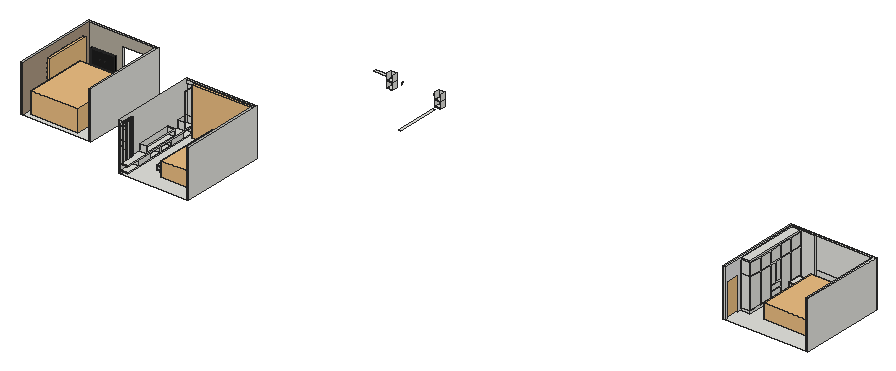
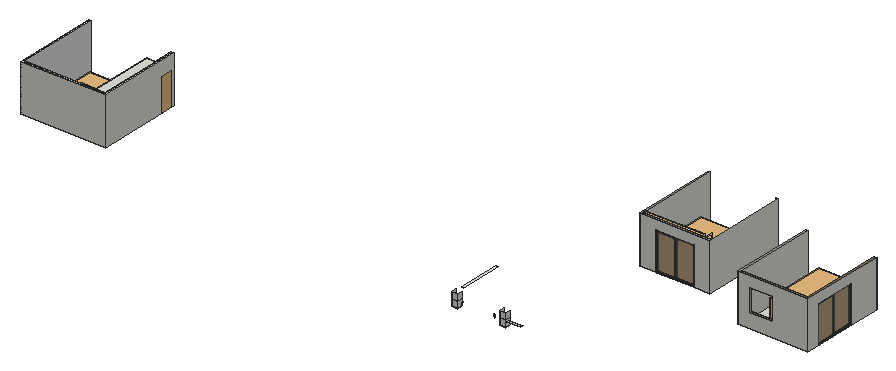
# SketchUp Ruby script. Lengths in inches.
U = 1.inch
M = Sketchup.active_model
def pt(a) = Geom::Point3d.new(a.map { |v| v * U })
def face(e, loops, mat)
  f = e.add_face(loops[0].map { |a| pt(a) })
  loops[1..].each { |l| e.add_face(l.map { |a| pt(a) }).erase! }
  f.material = f.back_material = mat if mat
  f
end
# faces: each face lists its corners as indices into pts; further lists are holes
def faces(e, pts, list, mat = nil) = list.each { |f| face(e, (f[0].is_a?(Array) ? f : [f]).map { |l| l.map { |i| pts[i] } }, mat) }
# xy, xz, yz: faces in a plane at the given z, y or x. An outline is a flat list of corners, or four numbers for a rectangle; further outlines are holes
def ring(l) = l.size == 4 ? [[l[0], l[1]], [l[2], l[1]], [l[2], l[3]], [l[0], l[3]]] : l.each_slice(2).to_a
def flat(e, list, mat, &to3) = list.each { |f| face(e, (f[0].is_a?(Array) ? f : [f]).map { |l| ring(l).map { |u, v| to3.(u, v) } }, mat) }
def xy(e, z, list, mat = nil) = flat(e, list, mat) { |x, y| [x, y, z] }
def xz(e, y, list, mat = nil) = flat(e, list, mat) { |x, z| [x, y, z] }
def yz(e, x, list, mat = nil) = flat(e, list, mat) { |y, z| [x, y, z] }
def lines(e, pts, list) = list.each { |a, b| e.add_line(pt(pts[a]), pt(pts[b])) }
# prism: a flat outline (further loops are holes) pulled along v
def prism(e, loops, v, mat = nil)
  f = face(e, loops, mat); d = Geom::Vector3d.new(v.map { |x| x * U })
  f.pushpull(f.normal.samedirection?(d) ? d.length : -d.length)
end
def box(e, o, s, mat = nil) = prism(e, [[o, [o[0] + s[0], o[1], o[2]], [o[0] + s[0], o[1] + s[1], o[2]], [o[0], o[1] + s[1], o[2]]]], [0, 0, s[2]], mat)
def at(x, y, z, deg = 0) = Geom::Transformation.translation(pt([x, y, z])) * Geom::Transformation.rotation(ORIGIN, Z_AXIS, deg.degrees)
def axes(o, x, y, z) = Geom::Transformation.new([*x, 0, *y, 0, *z, 0, *pt(o).to_a, 1])
def part(name) = M.definitions.add(name)
# library, detail: a bought-in or finely detailed component or shape, given as its bounding box
def library(name, o, s) = part(name).tap { |d| box(d.entities, o, s) }
def detail(e, o, s) = box(e.add_group.entities, o, s)
def put(e, d, t, mat = nil) = e.add_instance(d, t).tap { |i| i.material = mat if mat }
def group(e, t, mat = nil) = e.add_group.tap { |g| g.transformation = t; g.material = mat if mat }.entities
root = M.entities
M.materials.add("[0135_DarkGray]").color = [81, 81, 81]
M.materials.add("[Color_001]").color = [226, 226, 226]
M.materials.add("[Color_007]").color = [58, 58, 58]
M.materials.add("[Color_009]").color = [0, 0, 0]
M.materials.add("[Color_B19]").color = [180, 172, 158]
M.materials.add("[Color_D14]").color = [173, 154, 131]
M.materials.add("[Translucent Glass Gray]").color = [128, 128, 128]
M.materials["[Translucent Glass Gray]"].alpha = 0.15
M.materials.add("blackened steel1").color = [30, 30, 30]
c1 = library("bed",[-25.65,-58.99,0],[75.48,89.46,37.24])
c2 = library("Garniza_zaclona\#2",[1.52,0,0],[127.96,8.15,78.72])
c3 = part("PENTEK_RP Fineline 50S_SlidingDoor_GlazingBead_2")
box(c3.entities,[0,0,0],[0.56,0.59,94.39],"[0135_DarkGray]")
c4 = part("PENTEK_RP Fineline 50S_SlidingDoor_Glass")
box(c4.entities,[0,0,0],[46.58,0.16,94.39],"[Translucent Glass Gray]")
c5 = part("PENTEK_RP Fineline 50S_SlidingDoor_GlazingBead")
box(c5.entities,[0,0,0],[45.47,0.59,0.56],"[0135_DarkGray]")
c6 = part("PENTEK_RP Fineline 50S_SlidingDoor_Leaf_E1")
xy(c6.entities,0,[[0,0,0.93,1.97],[0.93,1.57,1.49,1.97]],"[0135_DarkGray]")
xy(c6.entities,96.25,[[0,0,0.93,0,0.93,1.57,1.49,1.57,1.49,1.97,0,1.97]],"[0135_DarkGray]")
xz(c6.entities,0,[[0,0,0.93,96.25]],"[0135_DarkGray]")
xz(c6.entities,1.57,[[0.93,0,1.49,95.32],[0.93,95.32,1.49,96.25]],"[0135_DarkGray]")
xz(c6.entities,1.97,[[0,0,1.49,96.25]],"[0135_DarkGray]")
yz(c6.entities,0,[[0,0,1.97,96.25]],"[0135_DarkGray]")
yz(c6.entities,0.93,[[0,0,1.57,0.93],[0,0.93,1.57,95.32],[0,95.32,1.57,96.25]],"[0135_DarkGray]")
yz(c6.entities,1.49,[[1.57,0,1.97,95.32],[1.57,95.32,1.97,96.25]],"[0135_DarkGray]")
c7 = part("PENTEK_RP Fineline 50S_SlidingDoor_Leaf_E2")
xy(c7.entities,0,[[0,0,0,1.57,0.56,1.57,0.56,1.97,46.02,1.97,46.02,1.57,46.58,1.57,46.58,0]],"[0135_DarkGray]")
xy(c7.entities,0.93,[[0,0,46.58,1.57]],"[0135_DarkGray]")
xy(c7.entities,1.49,[[0.56,1.57,46.02,1.97]],"[0135_DarkGray]")
xz(c7.entities,0,[[0,0,46.58,0.93]],"[0135_DarkGray]")
xz(c7.entities,1.57,[[0,0,0.56,0.93],[46.02,0,46.58,0.93],[0.56,0.93,46.02,1.49]],"[0135_DarkGray]")
xz(c7.entities,1.97,[[0.56,0,46.02,1.49]],"[0135_DarkGray]")
yz(c7.entities,0,[[0,0,1.57,0.93]],"[0135_DarkGray]")
yz(c7.entities,0.56,[[1.57,0,1.97,0.93],[1.57,0.93,1.97,1.49]],"[0135_DarkGray]")
yz(c7.entities,46.02,[[1.57,0,1.97,0.93],[1.57,0.93,1.97,1.49]],"[0135_DarkGray]")
yz(c7.entities,46.58,[[0,0,1.57,0.93]],"[0135_DarkGray]")
c8 = part("PENTEK_RP Fineline S_SlidingDoor_Leaf1")
put(c8.entities,c3,at(0.93,0,0.93))
put(c8.entities,c3,at(46.96,0,0.93))
put(c8.entities,c4,at(1.49,1.42,0.93))
put(c8.entities,c5,at(1.49,0,0.93))
put(c8.entities,c4,at(1.49,0.59,0.93))
put(c8.entities,c6,at(0,0,0))
put(c8.entities,c6,axes([48.44,0,0],[-1,0,0],[0,1,0],[0,0,1]))
put(c8.entities,c7,axes([0.93,0,96.25],[1,0,0],[0,1,0],[0,0,-1]))
put(c8.entities,c7,at(0.93,0,0))
put(c8.entities,c5,at(1.49,0,94.77))
c9 = part("PENTEK_RP Fineline 50S_Sliding_DoorCase_E1")
box(c9.entities,[0,0,0],[1.51,3.66,99.27],"[0135_DarkGray]")
c10 = part("PENTEK_RP Fineline 50S_SlidingDooe_Case_E2")
box(c10.entities,[0,0,0],[96.25,3.66,1.51],"[0135_DarkGray]")
c11 = part("pentek_RP Fineline 50S_SlidingDoor_Case")
put(c11.entities,c9,at(97.76,0,0))
put(c11.entities,c10,at(1.51,0,0))
put(c11.entities,c9,at(0,0,0))
put(c11.entities,c10,at(1.51,0,97.76))
c12 = part("PENTEK_RP Fineline 50S_SlidingDoor_Leaf2")
put(c12.entities,c4,at(1.49,1.42,0.93))
put(c12.entities,c5,at(1.49,0,94.77))
put(c12.entities,c3,at(46.96,0,0.93))
put(c12.entities,c4,at(1.49,0.59,0.93))
put(c12.entities,c3,at(0.93,0,0.93))
put(c12.entities,c6,at(0,0,0))
put(c12.entities,c6,axes([48.44,0,0],[-1,0,0],[0,1,0],[0,0,1]))
put(c12.entities,c5,at(1.49,0,0.93))
put(c12.entities,c7,axes([0.93,0,96.25],[1,0,0],[0,1,0],[0,0,-1]))
put(c12.entities,c7,at(0.93,0,0))
c13 = library("04+Sofa+y+Mesas",[-94.93,-111.67,3.93],[153.81,110.61,64.28])
c14 = library("Garniza_zaclona",[1.52,0,0],[127.96,8.15,78.72])
c15 = library("2222",[-1.18,-2.36,0],[68.11,146.45,38.04])
c16 = library("main+door",[0,-0.79,0],[47.24,7.88,82.68])
c17 = part("Vertical batten")
box(c17.entities,[0,0,0],[1,1,90])
xy(root,0,[[305.13,337.45,473.13,337.45,473.13,547.45,437.13,547.45,437.13,553.45,341.13,553.45,341.13,547.45,305.13,547.45],[174,400.17,180,400.17,180,616.17,0,616.17,0,586.17,6,586.17,6,592.17,174,592.17],[6,400.17,174,400.17,174,592.17,6,592.17,6,586.17,0,586.17,0,478.17,6,478.17],[1611.15,625.74,1815.15,625.74,1815.15,835.74,1671.15,835.74,1671.15,834.74,1635.15,834.74,1635.15,673.74,1611.15,673.74,1611.15,665.74,1605.15,665.74,1605.15,629.74,1611.15,629.74],[1635.15,834.74,1671.15,835.74]])
xy(root,1,[[7,592.17,33,592.35],[33,592.17,89,592.35],[90,592.17,110.5,609.17],[111.5,592.17,131.5,609.17],[132.5,592.17,152.5,609.17],
  [153.5,592.17,172.84,609.17]])
xy(root,1.2,[[7.2,592.17,33,592.35],[33,592.17,33.8,592.35],[34.2,592.17,35,592.35],[35,592.17,61.8,592.35],[62.2,592.17,88.8,592.35]])
xy(root,6,[[305.13,337.45,323.13,547.45],[1611.15,673.74,1635.15,835.74]])
xy(root,8,[[305.13,337.45,323.13,372.12],[305.13,510.78,323.13,545.45]])
xy(root,9,[[305.13,407.78,323.13,440.45],[305.13,442.45,323.13,475.12]])
xy(root,11.5,[[90,592.17,110.5,609.17],[111.5,592.17,131.5,609.17],[132.5,592.17,152.5,609.17],[153.5,592.17,172.84,609.17]])
xy(root,12.5,[[90,592.17,110.5,609.17],[111.5,592.17,131.5,609.17],[132.5,592.17,152.5,609.17],[153.5,592.17,172.84,609.17]])
xy(root,13.05,[[515.52,920.04,531.52,932.04],[637.52,920.04,653.52,932.04]])
xy(root,14.05,[[515.52,920.04,531.52,932.04],[637.52,920.04,653.52,932.04]])
xy(root,21,[[305.13,407.78,323.13,440.45],[305.13,442.45,323.13,475.12]])
xy(root,22,[[305.13,337.45,323.13,372.12],[305.13,510.78,323.13,545.45]])
xy(root,22.8,[[7.2,592.17,33.8,592.35],[34.2,592.17,61.8,592.35],[62.2,592.17,88.8,592.35]])
xy(root,23,[[7,592.17,33,592.35],[33,592.17,89,592.35],[90,592.17,110.5,609.17],[111.5,592.17,131.5,609.17],[132.5,592.17,152.5,609.17],
  [153.5,592.17,172.84,609.17]])
xy(root,24,[[305.13,337.45,323.13,397.45],[305.13,487.45,323.13,517.45],[6,592.17,174,610.17]])
xy(root,25,[[305.13,518.45,323.13,546.45]])
xy(root,26,[[305.13,399.45,323.13,485.45]])
xy(root,29.45,[[515.52,920.04,531.52,932.04],[637.52,920.04,653.52,932.04]])
xy(root,30.45,[[515.52,920.04,531.52,932.04],[637.52,920.04,653.52,932.04]])
xy(root,31.35,[[660.52,776.04,666.52,884.48],[472.52,932.04,508.52,938.04]])
xy(root,84,[[1605.15,629.74,1611.15,665.74]],"[Color_001]")
xy(root,116,[[1611.15,673.74,1635.15,835.74]])
xy(root,120,[[1605.15,625.74,1611.15,625.74,1611.15,835.74,1815.15,835.74,1815.15,625.74,1821.15,625.74,1821.15,841.74,1605.15,841.74],[1611.15,673.74,1635.15,835.74],[1635.15,834.74,1671.15,835.74]])
xz(root,337.45,[[299.13,0,305.13,0,305.13,6,323.13,6,323.13,8,305.13,8,305.13,22,323.13,22,323.13,24,305.13,24,305.13,120,299.13,120],[473.13,0,479.13,120]])
xz(root,372.12,[[305.13,8,323.13,22]])
xz(root,397.45,[[305.13,24,323.13,42]])
xz(root,399.45,[[305.13,26,323.13,40]])
xz(root,400.17,[[0,0,6,120],[174,0,180,120]])
xz(root,407.78,[[305.13,9,323.13,21]])
xz(root,440.45,[[305.13,9,323.13,21]])
xz(root,442.45,[[305.13,9,323.13,21]])
xz(root,475.12,[[305.13,9,323.13,21]])
xz(root,478.17,[[0,0,6,96]])
xz(root,485.45,[[305.13,26,323.13,40]])
xz(root,487.45,[[305.13,24,323.13,42]])
xz(root,510.78,[[305.13,8,323.13,22]])
xz(root,517.45,[[305.13,24,323.13,42]])
xz(root,518.45,[[305.13,25,323.13,41.5]])
xz(root,545.45,[[305.13,8,323.13,22]])
xz(root,546.45,[[305.13,25,323.13,41.5]])
xz(root,547.45,[[305.13,0,341.13,0,341.13,96,437.13,96,437.13,0,473.13,0,473.13,120,305.13,120,305.13,114,323.13,114,323.13,6,305.13,6]])
xz(root,553.45,[[299.13,0,299.13,120,479.13,120,479.13,0,437.13,0,437.13,96,341.13,96,341.13,0]])
xz(root,586.17,[[0,0,6,96]])
xz(root,592.17,[[[6,0,90,24],[7,1,89,23]],[90,0,132,1],[132,0,153,1],[153,0,174,0,174,11.5,172.84,11.5,172.84,1,153,1],[110.5,1,111.5,11.5],
  [131.5,1,132.5,11.5],[152.5,1,153.5,11.5],[7.2,1.2,33.8,22.8],[34.2,1.2,61.8,22.8],[62.2,1.2,88.8,22.8],
  [90,11.5,172.84,12.5],[172.84,11.5,174,12.5],[172.84,12.5,174,12.5,174,24,90,24,90,23,172.84,23],[110.5,12.5,111.5,23],[131.5,12.5,132.5,23],
  [152.5,12.5,153.5,23]])
xz(root,592.35,[[[7,1,89,23],[34.2,1.2,61.8,22.8],[62.2,1.2,88.8,22.8],[7.2,1.2,33.8,22.8]]])
xz(root,609.17,[[90,1,110.5,11.5],[111.5,1,131.5,11.5],[132.5,1,152.5,11.5],[153.5,1,172.84,11.5],[90,12.5,110.5,23],
  [111.5,12.5,131.5,23],[132.5,12.5,152.5,23],[153.5,12.5,172.84,23]])
xz(root,610.17,[[[6,24,174,120],[90,36,150,96]]],"[Color_B19]")
xz(root,616.17,[[[0,0,180,120],[90,36,150,96]]])
xz(root,625.74,[[1605.15,0,1611.15,120],[1815.15,0,1821.15,120]])
xz(root,629.74,[[1605.15,0,1611.15,84]])
xz(root,665.74,[[1605.15,0,1611.15,84]],"[Color_001]")
xz(root,673.74,[[1611.15,0,1635.15,6],[1611.15,6,1635.15,84],[1611.15,84,1635.15,116],[1611.15,116,1635.15,120]])
xz(root,834.74,[[1635.15,0,1671.15,120]])
xz(root,835.74,[[1635.15,0,1671.15,120],[1671.15,0,1815.15,42],[1611.15,6,1635.15,84],[1671.15,42,1815.15,120],[1611.15,84,1635.15,116],
  [1611.15,116,1635.15,120]])
xz(root,841.74,[[1605.15,0,1821.15,120]])
xz(root,920.04,[[515.52,13.05,531.52,14.05],[637.52,13.05,653.52,14.05],[515.52,29.45,531.52,30.45],[637.52,29.45,653.52,30.45]])
xz(root,932.04,[[515.52,14.05,531.52,29.45],[637.52,14.05,653.52,29.45],[515.52,30.45,531.52,46.35],[637.52,30.45,653.52,46.35]])
yz(root,0,[[400.17,0,400.17,120,616.17,120,616.17,0,586.17,0,586.17,96,478.17,96,478.17,0]])
yz(root,6,[[400.17,0,478.17,0,478.17,96,586.17,96,586.17,0,592.17,0,592.17,24,610.17,24,610.17,120,400.17,120]],"[Color_D14]")
yz(root,7,[[592.17,1,592.35,23]])
yz(root,7.2,[[592.17,1.2,592.35,22.8]])
yz(root,33.8,[[592.17,1.2,592.35,22.8]])
yz(root,34.2,[[592.17,1.2,592.35,22.8]])
yz(root,61.8,[[592.17,1.2,592.35,22.8]])
yz(root,62.2,[[592.17,1.2,592.35,22.8]])
yz(root,88.8,[[592.17,1.2,592.35,22.8]])
yz(root,89,[[592.17,1,592.35,23]])
yz(root,90,[[592.17,1,609.17,11.5],[592.17,12.5,609.17,23]])
yz(root,110.5,[[592.17,1,609.17,11.5],[592.17,12.5,609.17,23]])
yz(root,111.5,[[592.17,1,609.17,11.5],[592.17,12.5,609.17,23]])
yz(root,131.5,[[592.17,1,609.17,11.5],[592.17,12.5,609.17,23]])
yz(root,132.5,[[592.17,1,609.17,11.5],[592.17,12.5,609.17,23]])
yz(root,152.5,[[592.17,1,609.17,11.5],[592.17,12.5,609.17,23]])
yz(root,153.5,[[592.17,1,609.17,11.5],[592.17,12.5,609.17,23]])
yz(root,172.84,[[592.17,1,609.17,11.5],[592.17,12.5,609.17,23]])
yz(root,174,[[400.17,0,400.17,120,610.17,120,610.17,24,592.17,24,592.17,0]])
yz(root,180,[[400.17,0,616.17,120]])
yz(root,299.13,[[337.45,0,553.45,120]])
yz(root,305.13,[[337.45,0,547.45,6],[337.45,8,372.12,22],[510.78,8,545.45,22],[407.78,9,440.45,21],[442.45,9,475.12,21],
  [337.45,24,338.45,114],[518.45,25,546.45,41.5],[399.45,26,485.45,40]])
yz(root,323.13,[[337.45,6,547.45,6,547.45,24,337.45,24,337.45,22,545.45,22,545.45,8,337.45,8],[372.12,8,406.78,22],[[406.78,8,441.45,22],[407.78,9,440.45,21]],[[441.45,8,476.12,22],[442.45,9,475.12,21]],[476.12,8,510.78,22],
  [[397.45,24,487.45,42],[399.45,26,485.45,40]],[[517.45,24,547.45,114],[518.45,25,546.45,113]]])
yz(root,341.13,[[547.45,0,553.45,96]])
yz(root,437.13,[[547.45,0,553.45,96]])
yz(root,473.13,[[337.45,0,547.45,120]])
yz(root,479.13,[[337.45,0,553.45,120]])
yz(root,515.52,[[920.04,14.05,932.04,29.45],[920.04,30.45,932.04,46.35]])
yz(root,531.52,[[920.04,14.05,932.04,29.45],[920.04,30.45,932.04,46.35]])
yz(root,637.52,[[920.04,14.05,932.04,29.45],[920.04,30.45,932.04,46.35]])
yz(root,653.52,[[920.04,14.05,932.04,29.45],[920.04,30.45,932.04,46.35]])
yz(root,1605.15,[[625.74,0,625.74,120,841.74,120,841.74,0,665.74,0,665.74,84,629.74,84,629.74,0]])
yz(root,1611.15,[[673.74,6,835.74,84],[673.74,84,835.74,116],[673.74,116,835.74,120]])
yz(root,1611.15,[[625.74,0,629.74,0,629.74,84,665.74,84,665.74,0,673.74,0,673.74,120,625.74,120]],"[Color_001]")
yz(root,1635.15,[[673.74,0,834.74,6],[834.74,0,835.74,6],[[673.74,6,834.74,6,834.74,6.2,803.54,6.2,803.54,83.8,834.74,83.8,834.74,84.2,803.54,84.2,803.54,115.8,834.74,115.8,834.74,116,673.74,116],[706.34,6.2,738.34,83.8],[673.94,6.2,705.94,83.8],[771.14,6.2,803.14,83.8],[706.34,84.2,738.34,115.8],[738.74,84.2,770.74,115.8],[673.94,84.2,705.94,115.8],[771.14,84.2,803.14,115.8],[754.94,36.2,770.74,83.8],[738.74,36.2,754.54,83.8],[738.74,6.2,770.74,20.8],[738.74,21.2,770.74,35.8]],[834.74,6,834.74,6.2,835.54,6.2,835.54,83.8,834.74,83.8,834.74,84,835.74,84,835.74,6],[673.94,6.2,705.94,83.8],
  [706.34,6.2,738.34,83.8],[738.74,6.2,770.74,20.8],[771.14,6.2,803.14,83.8],[803.54,6.2,834.74,83.8],[834.74,6.2,835.54,83.8],
  [738.74,21.2,770.74,35.8],[738.74,36.2,754.54,83.8],[754.94,36.2,770.74,83.8],[834.74,84,835.74,84,835.74,116,834.74,116,834.74,115.8,835.54,115.8,835.54,84.2,834.74,84.2],[673.94,84.2,705.94,115.8],
  [706.34,84.2,738.34,115.8],[738.74,84.2,770.74,115.8],[771.14,84.2,803.14,115.8],[803.54,84.2,834.74,115.8],[834.74,84.2,835.54,115.8],
  [673.74,116,834.74,120],[834.74,116,835.74,120]])
yz(root,1671.15,[[834.74,0,835.74,120]])
yz(root,1815.15,[[625.74,0,835.74,120]],"[Color_001]")
yz(root,1821.15,[[625.74,0,841.74,120]])
p = [[544.08,932.04,27.17],[543.98,932.04,25.6],[543.98,931.54,25.6],[544.08,931.54,27.17],[627.33,932.04,25.6],[627.23,932.04,27.17],
  [627.23,931.54,27.17],[627.33,931.54,25.6],[544.39,932.04,28.71],[544.39,931.54,28.71],[626.92,932.04,28.71],[626.92,931.54,28.71],
  [544.89,932.04,30.2],[544.89,931.54,30.2],[626.42,932.04,30.2],[626.42,931.54,30.2],[545.59,932.04,31.6],[545.59,931.54,31.6],
  [625.73,932.04,31.6],[625.73,931.54,31.6],[546.46,932.04,32.91],[546.46,931.54,32.91],[624.85,932.04,32.91],[624.85,931.54,32.91]]
faces(root,p,[[0,1,2,3],[4,5,6,7],[8,0,3,9],[5,10,11,6],[12,8,9,13],[10,14,15,11],[16,12,13,17],[14,18,19,15],
  [20,16,17,21],[18,22,23,19]])
put(root,c1,axes([1706.9,773.18,0],[1.442,0,0],[0,1.6789,0],[0,0,1]))
put(root,c2,axes([14.15,474.72,0],[0,0.89,0],[-1,0,0],[0,0,1.24]))
g1 = group(root,at(4.02,478.17,0))
put(g1,c8,axes([0,1.66,1.46],[0,1.1,0],[-0.66,0,0],[0,0,0.96704]))
put(g1,c11,axes([-0.26,0,0],[0,1.1,0],[-0.66,0,0],[0,0,0.96704]))
put(g1,c12,axes([-1.3,54.25,1.46],[0,1.1,0],[-0.66,0,0],[0,0,0.96704]))
put(root,c13,axes([15.49,509.6,-3.3],[0,1.0164,0],[-1.0752,0,0],[0,0,0.84]))
put(root,c14,axes([322.77,539.3,0],[1.18455,0,0],[0,1,0],[0,0,1.52445]))
g2 = group(root,at(400.37,379.13,18))
xy(g2,-18,[[-37.73,10.14,-32.98,14.89],[-9.04,10.14,-4.29,14.89],[-37.73,59.26,-32.98,64.01],[-9.04,59.26,-4.29,64.01]])
xy(g2,-12,[[[-41.25,6,0,69.1875],[-9.04,10.14,-4.29,14.89],[-37.73,10.14,-32.98,14.89],[-37.73,59.26,-32.98,64.01],[-9.04,59.26,-4.29,64.01]]])
xy(g2,-10,[[-39.25,6,-2,66.5625]])
xy(g2,-2,[[-39.25,6,-2,66.5625]])
xy(g2,0,[[-41.25,6,0,69.1875]])
xz(g2,6,[[[-41.25,-12,0,0],[-39.25,-10,-2,-2]]])
xz(g2,10.14,[[-37.73,-18,-32.98,-12],[-9.04,-18,-4.29,-12]])
xz(g2,14.89,[[-37.73,-18,-32.98,-12],[-9.04,-18,-4.29,-12]])
xz(g2,59.26,[[-37.73,-18,-32.98,-12],[-9.04,-18,-4.29,-12]])
xz(g2,64.01,[[-37.73,-18,-32.98,-12],[-9.04,-18,-4.29,-12]])
xz(g2,66.5625,[[-39.25,-10,-2,-2]])
xz(g2,69.1875,[[-41.25,-12,0,0]])
yz(g2,-41.25,[[6,-12,69.1875,0]])
yz(g2,-39.25,[[6,-10,66.5625,-2]])
yz(g2,-37.73,[[10.14,-18,14.89,-12],[59.26,-18,64.01,-12]])
yz(g2,-32.98,[[10.14,-18,14.89,-12],[59.26,-18,64.01,-12]])
yz(g2,-9.04,[[10.14,-18,14.89,-12],[59.26,-18,64.01,-12]])
yz(g2,-4.29,[[10.14,-18,14.89,-12],[59.26,-18,64.01,-12]])
yz(g2,-2,[[6,-10,66.5625,-2]])
yz(g2,0,[[6,-12,69.1875,0]])
put(root,c15,axes([463.13,538.67,0],[-1.28,0,0],[0,-1.13,0],[0,0,1]))
g3 = group(root,at(341.13,548.75,0))
put(g3,c8,axes([1.46,0,1.46],[0.96704,0,0],[0,1,0],[0,0,0.96704]))
put(g3,c12,axes([47.69,1.97,1.46],[0.96704,0,0],[0,1,0],[0,0,0.96704]))
put(g3,c11,axes([0,0.39,0],[0.96704,0,0],[0,1,0],[0,0,0.96704]))
g4 = group(root,at(1781.79,789.47,0))
xy(g4,0,[[0,3.21,31.72,36.5625]])
xy(g4,1.8,[[1.8,3.21,29.92,3.39]])
xy(g4,1.98,[[1.98,3.21,29.75,3.39]])
xy(g4,10.3125,[[1.98,3.21,29.75,3.39]])
xy(g4,10.67,[[1.98,3.21,29.75,3.39]])
xy(g4,19,[[1.98,3.21,29.75,3.39]])
xy(g4,19.18,[[1.8,3.21,29.92,3.39]])
xy(g4,20.98,[[0,3.21,31.72,36.5625]])
xz(g4,3.21,[[1.98,1.98,29.75,10.3125],[1.98,10.67,29.75,19]])
xz(g4,3.21,[[[0,0,31.72,20.98],[1.8,1.8,29.92,19.18]]],"[Color_007]")
xz(g4,3.39,[[[1.8,1.8,29.92,19.18],[1.98,1.98,29.75,10.3125],[1.98,10.67,29.75,19]]],"[Color_007]")
xz(g4,36.5625,[[0,0,31.72,20.98]])
yz(g4,0,[[3.21,0,36.5625,20.98]])
yz(g4,1.8,[[3.21,1.8,3.39,19.18]])
yz(g4,1.98,[[3.21,1.98,3.39,10.3125],[3.21,10.67,3.39,19]])
yz(g4,29.75,[[3.21,1.98,3.39,10.3125],[3.21,10.67,3.39,19]])
yz(g4,29.92,[[3.21,1.8,3.39,19.18]])
yz(g4,31.72,[[3.21,0,36.5625,20.98]])
g5 = group(root,at(1637.22,789.47,0))
xy(g5,0,[[0,3.21,31.73,36.5625]])
xy(g5,1.8,[[1.8,3.21,29.92,3.39]])
xy(g5,1.98,[[1.98,3.21,29.74,3.39]])
xy(g5,10.3125,[[1.98,3.21,29.74,3.39]])
xy(g5,10.67,[[1.98,3.21,29.74,3.39]])
xy(g5,19,[[1.98,3.21,29.74,3.39]])
xy(g5,19.18,[[1.8,3.21,29.92,3.39]])
xy(g5,20.98,[[0,3.21,31.73,36.5625]])
xz(g5,3.21,[[1.98,1.98,29.74,10.3125],[1.98,10.67,29.74,19]])
xz(g5,3.21,[[[0,0,31.73,20.98],[1.8,1.8,29.92,19.18]]],"[Color_007]")
xz(g5,3.39,[[[1.8,1.8,29.92,19.18],[1.98,1.98,29.74,10.3125],[1.98,10.67,29.74,19]]],"[Color_007]")
xz(g5,36.5625,[[0,0,31.73,20.98]])
yz(g5,0,[[3.21,0,36.5625,20.98]])
yz(g5,1.8,[[3.21,1.8,3.39,19.18]])
yz(g5,1.98,[[3.21,1.98,3.39,10.3125],[3.21,10.67,3.39,19]])
yz(g5,29.74,[[3.21,1.98,3.39,10.3125],[3.21,10.67,3.39,19]])
yz(g5,29.92,[[3.21,1.8,3.39,19.18]])
yz(g5,31.73,[[3.21,0,36.5625,20.98]])
put(root,c16,axes([1606.49,665.74,0],[0,-0.762,0],[0.28,0,0],[0,0,1.016]))
put(root,c17,at(305.13,337.45,24))
put(root,c17,at(305.13,338.65,24))
put(root,c17,at(305.13,339.85,24))
put(root,c17,at(305.13,341.05,24))
put(root,c17,at(305.13,342.25,24))
put(root,c17,at(305.13,343.45,24))
put(root,c17,at(305.13,344.65,24))
put(root,c17,at(305.13,345.85,24))
put(root,c17,at(305.13,347.05,24))
put(root,c17,at(305.13,348.25,24))
put(root,c17,at(305.13,349.45,24))
put(root,c17,at(305.13,350.65,24))
put(root,c17,at(305.13,351.85,24))
put(root,c17,at(305.13,353.05,24))
put(root,c17,at(305.13,354.25,24))
put(root,c17,at(305.13,355.45,24))
put(root,c17,at(305.13,356.65,24))
put(root,c17,at(305.13,357.85,24))
put(root,c17,at(305.13,359.05,24))
put(root,c17,at(305.13,360.25,24))
put(root,c17,at(305.13,361.45,24))
put(root,c17,at(305.13,362.65,24))
put(root,c17,at(305.13,363.85,24))
put(root,c17,at(305.13,365.05,24))
put(root,c17,at(305.13,366.25,24))
put(root,c17,at(305.13,367.45,24))
put(root,c17,at(305.13,368.65,24))
put(root,c17,at(305.13,369.85,24))
put(root,c17,at(305.13,371.05,24))
put(root,c17,at(305.13,372.25,24))
g6 = group(root,at(76.1,604.81,30.94),"[Color_009]")
xy(g6,0,[[-59.67,0,0,2]])
xy(g6,15.8,[[-39.07,2,-26.26,5]])
xy(g6,21.42,[[-39.07,2,-26.26,5]])
xy(g6,36.875,[[-59.67,0,0,2]])
xz(g6,0,[[-59.67,0,0,36.875]],"blackened steel1")
xz(g6,2,[[[-59.67,0,0,36.875],[-39.07,15.8,-26.26,21.42]]])
xz(g6,5,[[-39.07,15.8,-26.26,21.42]])
yz(g6,-59.67,[[0,0,2,36.875]])
yz(g6,-39.07,[[2,15.8,5,21.42]])
yz(g6,-26.26,[[2,15.8,5,21.42]])
yz(g6,0,[[0,0,2,36.875]])
